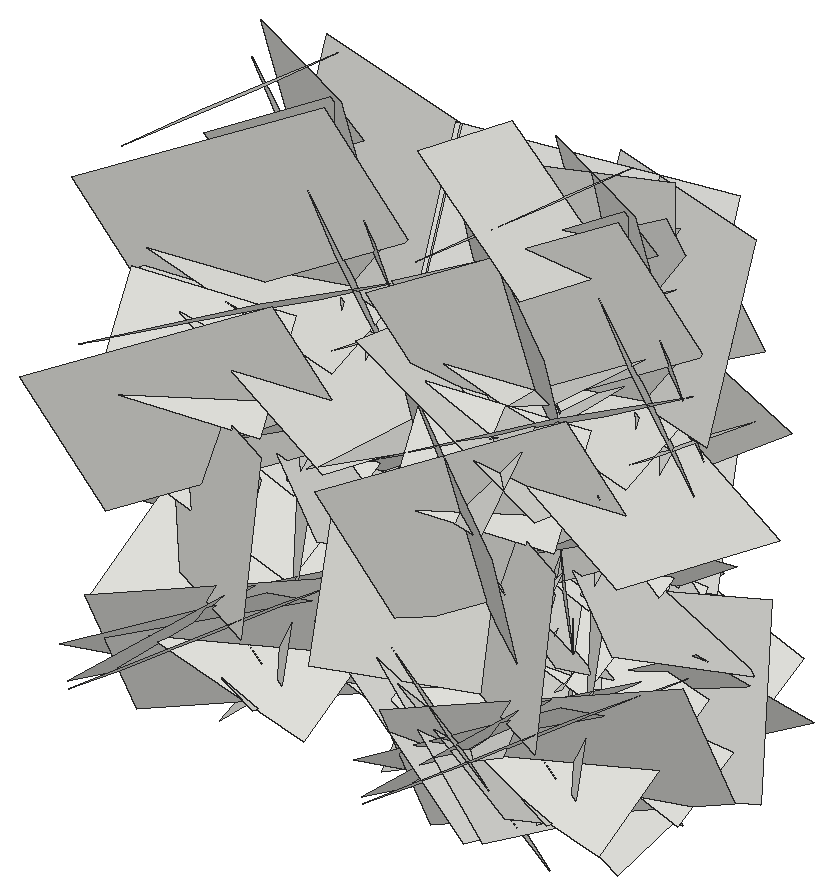
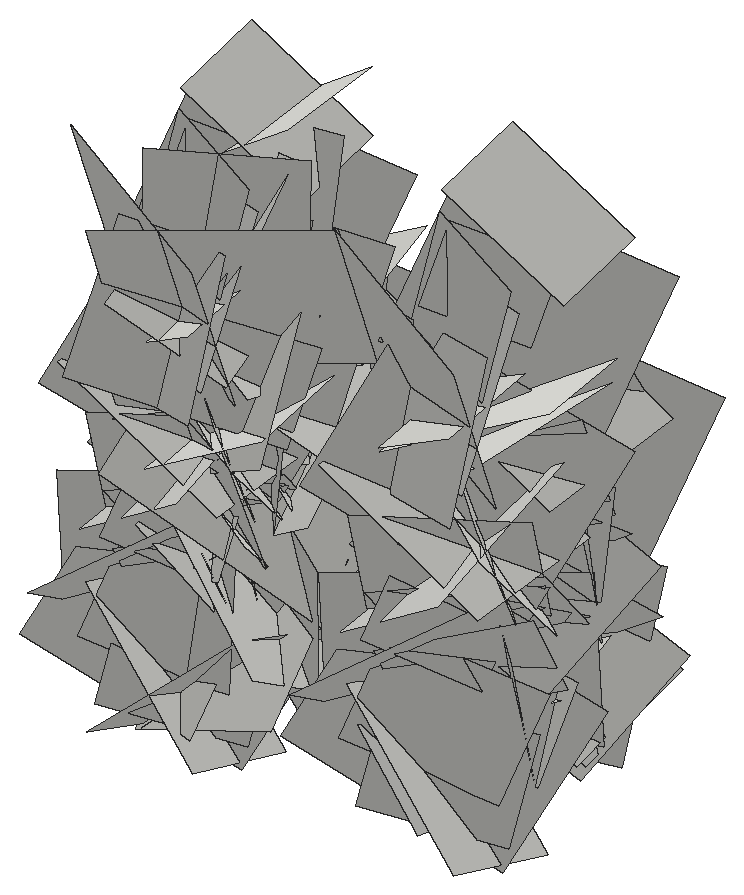
# SketchUp Ruby script. Lengths in inches.
U = 1.inch
M = Sketchup.active_model
def pt(a) = Geom::Point3d.new(a.map { |v| v * U })
def face(e, loops, mat)
  f = e.add_face(loops[0].map { |a| pt(a) })
  loops[1..].each { |l| e.add_face(l.map { |a| pt(a) }).erase! }
  f.material = f.back_material = mat if mat
  f
end
# faces: each face lists its corners as indices into pts; further lists are holes
def faces(e, pts, list, mat = nil) = list.each { |f| face(e, (f[0].is_a?(Array) ? f : [f]).map { |l| l.map { |i| pts[i] } }, mat) }
# xy, xz, yz: faces in a plane at the given z, y or x. An outline is a flat list of corners, or four numbers for a rectangle; further outlines are holes
def ring(l) = l.size == 4 ? [[l[0], l[1]], [l[2], l[1]], [l[2], l[3]], [l[0], l[3]]] : l.each_slice(2).to_a
def flat(e, list, mat, &to3) = list.each { |f| face(e, (f[0].is_a?(Array) ? f : [f]).map { |l| ring(l).map { |u, v| to3.(u, v) } }, mat) }
def xy(e, z, list, mat = nil) = flat(e, list, mat) { |x, y| [x, y, z] }
def xz(e, y, list, mat = nil) = flat(e, list, mat) { |x, z| [x, y, z] }
def yz(e, x, list, mat = nil) = flat(e, list, mat) { |y, z| [x, y, z] }
def lines(e, pts, list) = list.each { |a, b| e.add_line(pt(pts[a]), pt(pts[b])) }
# prism: a flat outline (further loops are holes) pulled along v
def prism(e, loops, v, mat = nil)
  f = face(e, loops, mat); d = Geom::Vector3d.new(v.map { |x| x * U })
  f.pushpull(f.normal.samedirection?(d) ? d.length : -d.length)
end
def box(e, o, s, mat = nil) = prism(e, [[o, [o[0] + s[0], o[1], o[2]], [o[0] + s[0], o[1] + s[1], o[2]], [o[0], o[1] + s[1], o[2]]]], [0, 0, s[2]], mat)
def at(x, y, z, deg = 0) = Geom::Transformation.translation(pt([x, y, z])) * Geom::Transformation.rotation(ORIGIN, Z_AXIS, deg.degrees)
def axes(o, x, y, z) = Geom::Transformation.new([*x, 0, *y, 0, *z, 0, *pt(o).to_a, 1])
def part(name) = M.definitions.add(name)
# library, detail: a bought-in or finely detailed component or shape, given as its bounding box
def library(name, o, s) = part(name).tap { |d| box(d.entities, o, s) }
def detail(e, o, s) = box(e.add_group.entities, o, s)
def put(e, d, t, mat = nil) = e.add_instance(d, t).tap { |i| i.material = mat if mat }
def group(e, t, mat = nil) = e.add_group.tap { |g| g.transformation = t; g.material = mat if mat }.entities
root = M.entities
c1 = part("Component\#6")
p = [[0.01,0,0],[0,3.24,4.54],[4.32,3.24,4.54],[4.33,0,0]]
faces(c1.entities,p,[[0,1,2,3]])
put(root,c1,axes([24.34,131.21,27.63],[-0.2234,-0.54463,1.08834],[-0.02633,1.10624,0.54877],[1.28976,-0.07175,0.19972]))
put(root,c1,axes([38.11,131.21,27.63],[0.2234,-0.54463,1.08834],[0.02633,1.10624,0.54877],[-1.28976,-0.07175,0.19972]))
put(root,c1,axes([34.14,131.21,27.63],[-0.2234,-0.54463,1.08834],[-0.02633,1.10624,0.54877],[1.28976,-0.07175,0.19972]))
put(root,c1,axes([24.34,134.27,30.6],[0.0256,-0.22889,-1.14247],[0.00761,-1.14266,0.22909],[1.23506,0.01178,0.02227]))
put(root,c1,axes([34.14,134.27,30.6],[0.0256,-0.22889,-1.14247],[0.00761,-1.14266,0.22909],[1.23506,0.01178,0.02227]))
put(root,c1,axes([38.11,134.27,30.6],[-0.0256,-0.22889,-1.14247],[-0.00761,-1.14266,0.22909],[-1.23506,0.01178,0.02227]))
put(root,c1,axes([34.14,134.18,33.55],[-0.07538,-0.44425,-0.62436],[0.04133,-0.62833,0.44263],[0.8112,-0.00926,-0.08057]))
put(root,c1,axes([28.31,134.18,33.55],[0.07538,-0.44425,-0.62436],[-0.04133,-0.62833,0.44263],[-0.8112,-0.00926,-0.08057]))
put(root,c1,axes([38.11,134.18,33.55],[0.07538,-0.44425,-0.62436],[-0.04133,-0.62833,0.44263],[-0.8112,-0.00926,-0.08057]))
put(root,c1,axes([24.34,134.17,21.91],[-0.00769,-1.04417,0.30366],[-0.13881,0.30229,1.03635],[1.14428,0.02965,0.12776]))
put(root,c1,axes([34.14,134.17,21.91],[-0.00769,-1.04417,0.30366],[-0.13881,0.30229,1.03635],[1.14428,0.02965,0.12776]))
put(root,c1,axes([38.11,134.17,21.91],[0.00769,-1.04417,0.30366],[0.13881,0.30229,1.03635],[-1.14428,0.02965,0.12776]))
put(root,c1,axes([24.34,134.58,22.11],[0.07114,-1.22092,0.271],[-0.02912,0.26988,1.2227],[1.32535,0.07146,0.01232]))
put(root,c1,axes([38.11,134.58,22.11],[-0.07114,-1.22092,0.271],[0.02912,0.26988,1.2227],[-1.32535,0.07146,0.01232]))
put(root,c1,axes([34.14,134.58,22.11],[0.07114,-1.22092,0.271],[-0.02912,0.26988,1.2227],[1.32535,0.07146,0.01232]))
put(root,c1,axes([24.34,134.42,21.5625],[-0.1234,-1.02964,0.56694],[0.11588,0.55776,1.03542],[1.24053,-0.15452,-0.04032]))
put(root,c1,axes([34.14,134.42,21.5625],[-0.1234,-1.02964,0.56694],[0.11588,0.55776,1.03542],[1.24053,-0.15452,-0.04032]))
put(root,c1,axes([38.11,134.42,21.5625],[0.1234,-1.02964,0.56694],[-0.11588,0.55776,1.03542],[-1.24053,-0.15452,-0.04032]))
put(root,c1,axes([24.34,132.49,21.15],[0.19066,-0.73145,1.17679],[0.11238,1.19045,0.72374],[1.46442,0.00387,-0.20876]))
put(root,c1,axes([34.14,132.49,21.15],[0.19066,-0.73145,1.17679],[0.11238,1.19045,0.72374],[1.46442,0.00387,-0.20876]))
put(root,c1,axes([38.11,132.49,21.15],[-0.19066,-0.73145,1.17679],[-0.11238,1.19045,0.72374],[-1.46442,0.00387,-0.20876]))
put(root,c1,axes([34.14,134.6875,22.2],[-0.10426,-0.66856,0.17597],[0.06243,0.169,0.67497],[0.73015,-0.10992,-0.03258]))
put(root,c1,axes([28.31,134.6875,22.2],[0.10426,-0.66856,0.17597],[-0.06243,0.169,0.67497],[-0.73015,-0.10992,-0.03258]))
put(root,c1,axes([38.11,134.6875,22.2],[0.10426,-0.66856,0.17597],[-0.06243,0.169,0.67497],[-0.73015,-0.10992,-0.03258]))
put(root,c1,axes([28.31,131.06,25.92],[0.11704,0.23417,0.88186],[0.10525,0.87993,-0.24609],[-0.96142,0.12483,0.08041]))
put(root,c1,axes([34.14,131.06,25.92],[-0.11704,0.23417,0.88186],[-0.10525,0.87993,-0.24609],[0.96142,0.12483,0.08041]))
put(root,c1,axes([38.11,131.06,25.92],[0.11704,0.23417,0.88186],[0.10525,0.87993,-0.24609],[-0.96142,0.12483,0.08041]))
put(root,c1,axes([24.34,130.54,25.39],[0.14552,0.87979,0.74939],[0.0105,0.75374,-0.8867],[1.22498,-0.11098,-0.08143]))
put(root,c1,axes([34.14,130.54,25.39],[0.14552,0.87979,0.74939],[0.0105,0.75374,-0.8867],[1.22498,-0.11098,-0.08143]))
put(root,c1,axes([38.11,130.54,25.39],[-0.14552,0.87979,0.74939],[-0.0105,0.75374,-0.8867],[-1.22498,-0.11098,-0.08143]))
put(root,c1,axes([24.34,135.84,31.22],[-0.16391,-1.12855,0.28901],[0.13375,0.27361,1.13591],[1.2276,-0.1805,-0.08517]))
put(root,c1,axes([34.14,135.84,31.22],[-0.16391,-1.12855,0.28901],[0.13375,0.27361,1.13591],[1.2276,-0.1805,-0.08517]))
put(root,c1,axes([38.11,135.84,31.22],[0.16391,-1.12855,0.28901],[-0.13375,0.27361,1.13591],[-1.2276,-0.1805,-0.08517]))
put(root,c1,axes([24.34,135.18,37.85],[0.05885,-0.83818,0.13983],[-0.03078,0.13818,0.83979],[0.90022,0.05952,0.01957]))
put(root,c1,axes([34.14,135.18,37.85],[0.05885,-0.83818,0.13983],[-0.03078,0.13818,0.83979],[0.90022,0.05952,0.01957]))
put(root,c1,axes([38.11,135.18,37.85],[-0.05885,-0.83818,0.13983],[0.03078,0.13818,0.83979],[-0.90022,0.05952,0.01957]))
put(root,c1,axes([24.34,133.37,32.625],[-0.2234,-0.54463,1.08834],[-0.02633,1.10624,0.54877],[1.28976,-0.07175,0.19972]))
put(root,c1,axes([38.11,133.37,32.625],[0.2234,-0.54463,1.08834],[0.02633,1.10624,0.54877],[-1.28976,-0.07175,0.19972]))
put(root,c1,axes([34.14,133.37,32.625],[-0.2234,-0.54463,1.08834],[-0.02633,1.10624,0.54877],[1.28976,-0.07175,0.19972]))
put(root,c1,axes([24.34,131.97,28.78],[0.10091,0.74431,0.53228],[-0.01265,0.53611,-0.74754],[0.96987,-0.07045,-0.06513]))
put(root,c1,axes([34.14,131.97,28.78],[0.10091,0.74431,0.53228],[-0.01265,0.53611,-0.74754],[0.96987,-0.07045,-0.06513]))
put(root,c1,axes([38.11,131.97,28.78],[-0.10091,0.74431,0.53228],[0.01265,0.53611,-0.74754],[-0.96987,-0.07045,-0.06513]))
put(root,c1,axes([28.31,136.41,29.65],[0.07813,-0.63244,-0.26103],[0.10098,-0.25049,0.63382],[-0.71818,-0.10402,0.06072]))
put(root,c1,axes([34.14,136.41,29.65],[-0.07813,-0.63244,-0.26103],[-0.10098,-0.25049,0.63382],[0.71818,-0.10402,0.06072]))
put(root,c1,axes([38.11,136.41,29.65],[0.07813,-0.63244,-0.26103],[0.10098,-0.25049,0.63382],[-0.71818,-0.10402,0.06072]))
put(root,c1,axes([24.34,134.54,24.9375],[0.02484,0.40022,-0.64969],[0.07983,-0.64803,-0.39648],[0.8049,0.05192,0.05937]))
put(root,c1,axes([34.14,134.54,24.9375],[0.02484,0.40022,-0.64969],[0.07983,-0.64803,-0.39648],[0.8049,0.05192,0.05937]))
put(root,c1,axes([38.11,134.54,24.9375],[-0.02484,0.40022,-0.64969],[-0.07983,-0.64803,-0.39648],[-0.8049,0.05192,0.05937]))
put(root,c1,axes([24.34,136.25,25.03],[-0.1909,-1.05424,0.65515],[0.04228,0.65676,1.06778],[1.31502,-0.17416,0.06077]))
put(root,c1,axes([34.14,136.25,25.03],[-0.1909,-1.05424,0.65515],[0.04228,0.65676,1.06778],[1.31502,-0.17416,0.06077]))
put(root,c1,axes([38.11,136.25,25.03],[0.1909,-1.05424,0.65515],[-0.04228,0.65676,1.06778],[-1.31502,-0.17416,0.06077]))
put(root,c1,axes([24.34,132.63,34.3],[0.186,1.33026,-0.17859],[0.24164,-0.20703,-1.31812],[1.40205,-0.1408,0.25087]))
put(root,c1,axes([34.14,132.63,34.3],[0.186,1.33026,-0.17859],[0.24164,-0.20703,-1.31812],[1.40205,-0.1408,0.25087]))
put(root,c1,axes([38.11,132.63,34.3],[-0.186,1.33026,-0.17859],[-0.24164,-0.20703,-1.31812],[-1.40205,-0.1408,0.25087]))
put(root,c1,axes([24.34,132.79,29.8],[0.04873,0.29435,0.84438],[-0.1159,0.841,-0.28722],[0.94075,0.08836,-0.07912]))
put(root,c1,axes([38.11,132.79,29.8],[-0.04873,0.29435,0.84438],[0.1159,0.841,-0.28722],[-0.94075,0.08836,-0.07912]))
put(root,c1,axes([34.14,132.79,29.8],[0.04873,0.29435,0.84438],[-0.1159,0.841,-0.28722],[0.94075,0.08836,-0.07912]))
put(root,c1,axes([24.34,137.68,26.93],[0.04018,-0.30696,-1.06119],[-0.15368,-1.05402,0.2997],[1.16085,-0.12891,0.07641]))
put(root,c1,axes([34.14,137.68,26.93],[0.04018,-0.30696,-1.06119],[-0.15368,-1.05402,0.2997],[1.16085,-0.12891,0.07641]))
put(root,c1,axes([38.11,137.68,26.93],[-0.04018,-0.30696,-1.06119],[0.15368,-1.05402,0.2997],[-1.16085,-0.12891,0.07641]))
put(root,c1,axes([24.34,133.57,26.39],[-0.0097,-0.16576,1.00827],[-0.11893,1.00238,0.16377],[1.07657,0.10924,0.02717]))
put(root,c1,axes([34.14,133.57,26.39],[-0.0097,-0.16576,1.00827],[-0.11893,1.00238,0.16377],[1.07657,0.10924,0.02717]))
put(root,c1,axes([38.11,133.57,26.39],[0.0097,-0.16576,1.00827],[0.11893,1.00238,0.16377],[-1.07657,0.10924,0.02717]))
put(root,c1,axes([34.14,135.55,39.48],[0.03347,0.37514,-0.47819],[-0.05412,-0.47551,-0.37641],[0.64197,-0.05964,-0.0068]))
put(root,c1,axes([28.31,135.55,39.48],[-0.03347,0.37514,-0.47819],[0.05412,-0.47551,-0.37641],[-0.64197,-0.05964,-0.0068]))
put(root,c1,axes([38.11,135.55,39.48],[-0.03347,0.37514,-0.47819],[0.05412,-0.47551,-0.37641],[-0.64197,-0.05964,-0.0068]))
put(root,c1,axes([24.34,132.63,35],[-0.22269,1.01925,0.0867],[0.15354,0.11726,-1.02752],[1.07338,0.19468,0.16497]))
put(root,c1,axes([34.14,132.63,35],[-0.22269,1.01925,0.0867],[0.15354,0.11726,-1.02752],[1.07338,0.19468,0.16497]))
put(root,c1,axes([38.11,132.63,35],[0.22269,1.01925,0.0867],[-0.15354,0.11726,-1.02752],[-1.07338,0.19468,0.16497]))
put(root,c1,axes([24.34,133.32,22.11],[0.03082,0.0656,1.39488],[-0.001,1.39518,-0.0656],[1.48021,-0.00042,-0.02909]))
put(root,c1,axes([34.14,133.32,22.11],[0.03082,0.0656,1.39488],[-0.001,1.39518,-0.0656],[1.48021,-0.00042,-0.02909]))
put(root,c1,axes([38.11,133.32,22.11],[-0.03082,0.0656,1.39488],[0.001,1.39518,-0.0656],[-1.48021,-0.00042,-0.02909]))
put(root,c1,axes([24.34,133.77,26.39],[-0.09062,0.64279,0.71838],[0.13606,0.72237,-0.63108],[1.01272,-0.03954,0.14907]))
put(root,c1,axes([34.14,133.77,26.39],[-0.09062,0.64279,0.71838],[0.13606,0.72237,-0.63108],[1.01272,-0.03954,0.14907]))
put(root,c1,axes([38.11,133.77,26.39],[0.09062,0.64279,0.71838],[-0.13606,0.72237,-0.63108],[-1.01272,-0.03954,0.14907]))
put(root,c1,axes([24.34,139.12,30.95],[-0.15428,-0.64193,-0.79007],[0.04846,-0.80142,0.64273],[1.07797,-0.05585,-0.14197]))
put(root,c1,axes([34.14,139.12,30.95],[-0.15428,-0.64193,-0.79007],[0.04846,-0.80142,0.64273],[1.07797,-0.05585,-0.14197]))
put(root,c1,axes([38.11,139.12,30.95],[0.15428,-0.64193,-0.79007],[-0.04846,-0.80142,0.64273],[-1.07797,-0.05585,-0.14197]))
put(root,c1,axes([24.34,134.64,27.51],[0.11331,0.92563,-0.03565],[-0.09128,-0.0258,-0.92812],[0.97764,-0.10969,-0.08252]))
put(root,c1,axes([34.14,134.64,27.51],[0.11331,0.92563,-0.03565],[-0.09128,-0.0258,-0.92812],[0.97764,-0.10969,-0.08252]))
put(root,c1,axes([38.11,134.64,27.51],[-0.11331,0.92563,-0.03565],[0.09128,-0.0258,-0.92812],[-0.97764,-0.10969,-0.08252]))
put(root,c1,axes([24.34,135.17,32.61],[0.12448,1.21649,-0.63228],[-0.14654,-0.62086,-1.22019],[1.44585,-0.16766,-0.06923]))
put(root,c1,axes([34.14,135.17,32.61],[0.12448,1.21649,-0.63228],[-0.14654,-0.62086,-1.22019],[1.44585,-0.16766,-0.06923]))
put(root,c1,axes([38.11,135.17,32.61],[-0.12448,1.21649,-0.63228],[0.14654,-0.62086,-1.22019],[-1.44585,-0.16766,-0.06923]))
put(root,c1,axes([24.34,136.8125,27.97],[-0.23976,-0.84366,1.03424],[-0.08712,1.0558,0.84327],[1.41209,-0.07811,0.22763]))
put(root,c1,axes([34.14,136.8125,27.97],[-0.23976,-0.84366,1.03424],[-0.08712,1.0558,0.84327],[1.41209,-0.07811,0.22763]))
put(root,c1,axes([38.11,136.8125,27.97],[0.23976,-0.84366,1.03424],[0.08712,1.0558,0.84327],[-1.41209,-0.07811,0.22763]))
put(root,c1,axes([24.34,132.97,26.35],[0.04012,1.17129,0.65858],[-0.12839,0.65914,-1.16531],[1.41857,0.02653,-0.1241]))
put(root,c1,axes([34.14,132.97,26.35],[0.04012,1.17129,0.65858],[-0.12839,0.65914,-1.16531],[1.41857,0.02653,-0.1241]))
put(root,c1,axes([38.11,132.97,26.35],[-0.04012,1.17129,0.65858],[0.12839,0.65914,-1.16531],[-1.41857,0.02653,-0.1241]))
put(root,c1,axes([24.34,137.29,38.52],[-0.00887,0.62519,-1.13199],[-0.07674,-1.13046,-0.62381],[1.3686,-0.05933,-0.04231]))
put(root,c1,axes([34.14,137.29,38.52],[-0.00887,0.62519,-1.13199],[-0.07674,-1.13046,-0.62381],[1.3686,-0.05933,-0.04231]))
put(root,c1,axes([38.11,137.29,38.52],[0.00887,0.62519,-1.13199],[0.07674,-1.13046,-0.62381],[-1.3686,-0.05933,-0.04231]))
put(root,c1,axes([28.31,134.33,29.51],[0.0444,0.3698,0.86525],[0.11423,0.85852,-0.37214],[-0.99086,0.11554,-0.00413]))
put(root,c1,axes([34.14,134.33,29.51],[-0.0444,0.3698,0.86525],[-0.11423,0.85852,-0.37214],[0.99086,0.11554,-0.00413]))
put(root,c1,axes([38.11,134.33,29.51],[0.0444,0.3698,0.86525],[0.11423,0.85852,-0.37214],[-0.99086,0.11554,-0.00413]))
put(root,c1,axes([24.34,139.23,29.07],[-0.06497,-1.13195,0.1646],[0.10003,0.15928,1.13044],[1.20835,-0.07404,-0.08473]))
put(root,c1,axes([34.14,139.23,29.07],[-0.06497,-1.13195,0.1646],[0.10003,0.15928,1.13044],[1.20835,-0.07404,-0.08473]))
put(root,c1,axes([38.11,139.23,29.07],[0.06497,-1.13195,0.1646],[-0.10003,0.15928,1.13044],[-1.20835,-0.07404,-0.08473]))
put(root,c1,axes([24.34,137.68,39.44],[0.12024,0.16456,-0.83242],[0.12638,-0.83458,-0.14874],[0.89051,0.09622,0.13351]))
put(root,c1,axes([34.14,137.68,39.44],[0.12024,0.16456,-0.83242],[0.12638,-0.83458,-0.14874],[0.89051,0.09622,0.13351]))
put(root,c1,axes([38.11,137.68,39.44],[-0.12024,0.16456,-0.83242],[-0.12638,-0.83458,-0.14874],[-0.89051,0.09622,0.13351]))
put(root,c1,axes([24.34,138.04,20.07],[-0.12016,-0.9858,0.86253],[0.12902,0.85408,0.99214],[1.38246,-0.16539,-0.01763]))
put(root,c1,axes([38.11,138.04,20.07],[0.12016,-0.9858,0.86253],[-0.12902,0.85408,0.99214],[-1.38246,-0.16539,-0.01763]))
put(root,c1,axes([34.14,138.04,20.07],[-0.12016,-0.9858,0.86253],[0.12902,0.85408,0.99214],[1.38246,-0.16539,-0.01763]))
put(root,c1,axes([34.14,139.13,26.61],[-0.02912,-0.4172,-0.72752],[-0.02466,-0.72725,0.41792],[0.88863,-0.03385,-0.01224]))
put(root,c1,axes([28.31,139.13,26.61],[0.02912,-0.4172,-0.72752],[0.02466,-0.72725,0.41792],[-0.88863,-0.03385,-0.01224]))
put(root,c1,axes([38.11,139.13,26.61],[0.02912,-0.4172,-0.72752],[0.02466,-0.72725,0.41792],[-0.88863,-0.03385,-0.01224]))
put(root,c1,axes([24.34,140.34,20.98],[0.05969,-1.08852,-0.33352],[-0.17093,-0.33819,1.07653],[1.19461,0.00599,0.1707]))
put(root,c1,axes([38.11,140.34,20.98],[-0.05969,-1.08852,-0.33352],[0.17093,-0.33819,1.07653],[-1.19461,0.00599,0.1707]))
put(root,c1,axes([34.14,140.34,20.98],[0.05969,-1.08852,-0.33352],[-0.17093,-0.33819,1.07653],[1.19461,0.00599,0.1707]))
put(root,c1,axes([34.14,137.74,29.49],[-0.05063,0.39266,-0.56355],[-0.15447,-0.55784,-0.37633],[0.71149,-0.09317,-0.12181]))
put(root,c1,axes([28.31,137.74,29.49],[0.05063,0.39266,-0.56355],[0.15447,-0.55784,-0.37633],[-0.71149,-0.09317,-0.12181]))
put(root,c1,axes([38.11,137.74,29.49],[0.05063,0.39266,-0.56355],[0.15447,-0.55784,-0.37633],[-0.71149,-0.09317,-0.12181]))
put(root,c1,axes([24.34,135.78,27.7],[-0.08438,0.31612,0.89331],[0.15155,0.8902,-0.30228],[0.99295,-0.109,0.12205]))
put(root,c1,axes([34.14,135.78,27.7],[-0.08438,0.31612,0.89331],[0.15155,0.8902,-0.30228],[0.99295,-0.109,0.12205]))
put(root,c1,axes([38.11,135.78,27.7],[0.08438,0.31612,0.89331],[-0.15155,0.8902,-0.30228],[-0.99295,-0.109,0.12205]))
put(root,c1,axes([24.34,140.4,37.84],[-0.00777,-0.46206,-1.23937],[0.21731,-1.22481,0.45542],[1.38512,0.18957,-0.0784]))
put(root,c1,axes([38.11,140.4,37.84],[0.00777,-0.46206,-1.23937],[-0.21731,-1.22481,0.45542],[-1.38512,0.18957,-0.0784]))
put(root,c1,axes([34.14,140.4,37.84],[-0.00777,-0.46206,-1.23937],[0.21731,-1.22481,0.45542],[1.38512,0.18957,-0.0784]))
put(root,c1,axes([34.14,138.35,27.1],[-0.19626,0.31166,-0.79897],[0.02742,-0.81497,-0.3239],[0.90864,0.09191,-0.1628]))
put(root,c1,axes([28.31,138.35,27.1],[0.19626,0.31166,-0.79897],[-0.02742,-0.81497,-0.3239],[-0.90864,0.09191,-0.1628]))
put(root,c1,axes([38.11,138.35,27.1],[0.19626,0.31166,-0.79897],[-0.02742,-0.81497,-0.3239],[-0.90864,0.09191,-0.1628]))
put(root,c1,axes([24.34,137.01,36.4],[0.10049,0.69541,-0.2411],[0.01368,-0.24463,-0.7005],[0.78006,-0.08529,0.04335]))
put(root,c1,axes([34.14,137.01,36.4],[0.10049,0.69541,-0.2411],[0.01368,-0.24463,-0.7005],[0.78006,-0.08529,0.04335]))
put(root,c1,axes([38.11,137.01,36.4],[-0.10049,0.69541,-0.2411],[-0.01368,-0.24463,-0.7005],[-0.78006,-0.08529,0.04335]))
put(root,c1,axes([24.34,137.76,20.74],[0.07875,-0.43706,0.66864],[-0.02301,0.67018,0.44047],[0.84643,0.05888,-0.05024]))
put(root,c1,axes([34.14,137.76,20.74],[0.07875,-0.43706,0.66864],[-0.02301,0.67018,0.44047],[0.84643,0.05888,-0.05024]))
put(root,c1,axes([38.11,137.76,20.74],[-0.07875,-0.43706,0.66864],[0.02301,0.67018,0.44047],[-0.84643,0.05888,-0.05024]))
put(root,c1,axes([24.34,138.81,37.71],[-0.08326,0.50336,-1.07522],[-0.02589,-1.07803,-0.50289],[1.25818,0.01113,-0.0815]))
put(root,c1,axes([34.14,138.81,37.71],[-0.08326,0.50336,-1.07522],[-0.02589,-1.07803,-0.50289],[1.25818,0.01113,-0.0815]))
put(root,c1,axes([38.11,138.81,37.71],[0.08326,0.50336,-1.07522],[0.02589,-1.07803,-0.50289],[-1.25818,0.01113,-0.0815]))
put(root,c1,axes([34.14,136.62,23.89],[-0.08859,0.63974,0.04756],[-0.12242,0.03217,-0.63572],[0.66888,0.09062,-0.11005]))
put(root,c1,axes([28.31,136.62,23.89],[0.08859,0.63974,0.04756],[0.12242,0.03217,-0.63572],[-0.66888,0.09062,-0.11005]))
